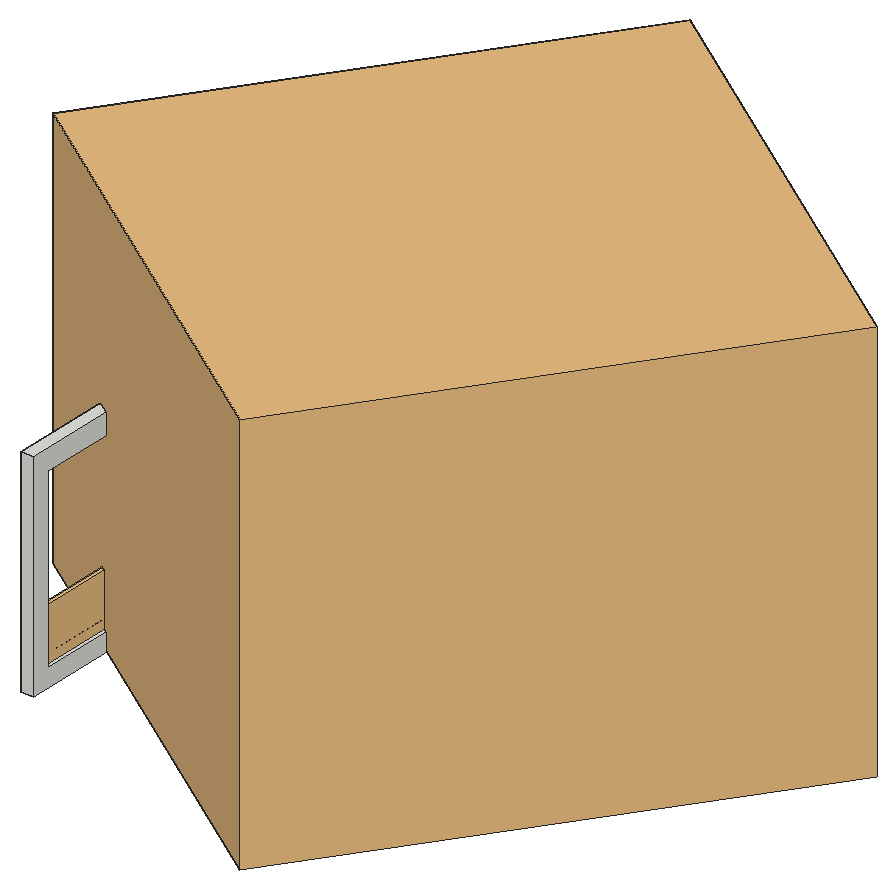
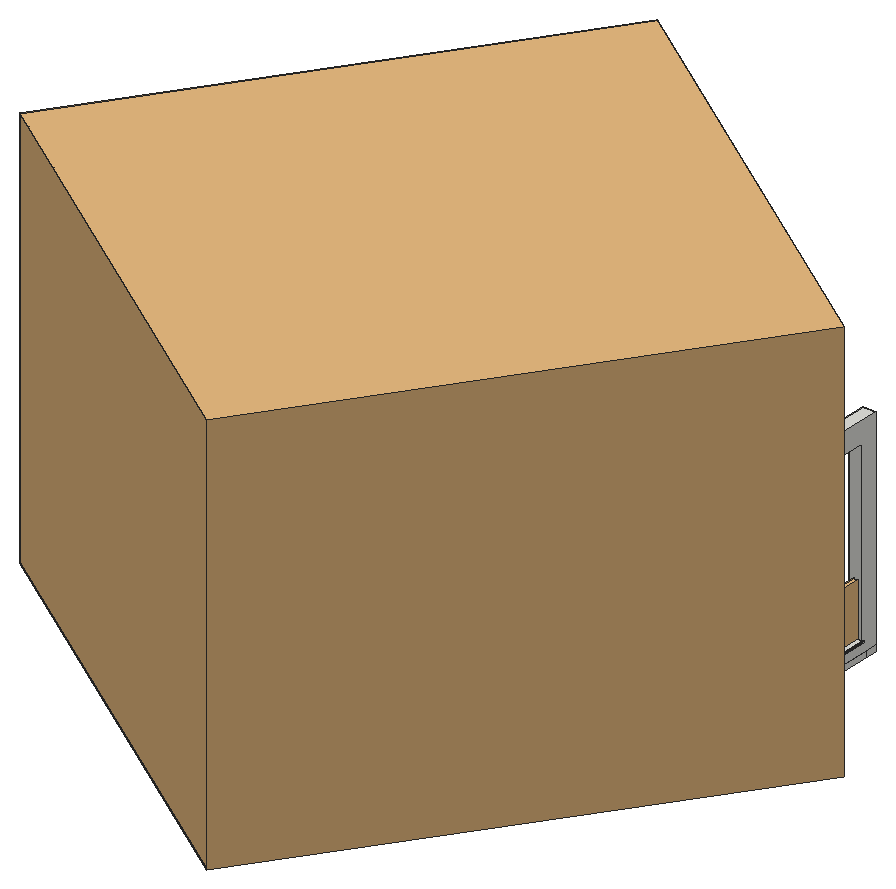
# SketchUp Ruby script. Lengths in inches.
U = 1.inch
M = Sketchup.active_model
def pt(a) = Geom::Point3d.new(a.map { |v| v * U })
def face(e, loops, mat)
  f = e.add_face(loops[0].map { |a| pt(a) })
  loops[1..].each { |l| e.add_face(l.map { |a| pt(a) }).erase! }
  f.material = f.back_material = mat if mat
  f
end
# faces: each face lists its corners as indices into pts; further lists are holes
def faces(e, pts, list, mat = nil) = list.each { |f| face(e, (f[0].is_a?(Array) ? f : [f]).map { |l| l.map { |i| pts[i] } }, mat) }
# xy, xz, yz: faces in a plane at the given z, y or x. An outline is a flat list of corners, or four numbers for a rectangle; further outlines are holes
def ring(l) = l.size == 4 ? [[l[0], l[1]], [l[2], l[1]], [l[2], l[3]], [l[0], l[3]]] : l.each_slice(2).to_a
def flat(e, list, mat, &to3) = list.each { |f| face(e, (f[0].is_a?(Array) ? f : [f]).map { |l| ring(l).map { |u, v| to3.(u, v) } }, mat) }
def xy(e, z, list, mat = nil) = flat(e, list, mat) { |x, y| [x, y, z] }
def xz(e, y, list, mat = nil) = flat(e, list, mat) { |x, z| [x, y, z] }
def yz(e, x, list, mat = nil) = flat(e, list, mat) { |y, z| [x, y, z] }
def lines(e, pts, list) = list.each { |a, b| e.add_line(pt(pts[a]), pt(pts[b])) }
# prism: a flat outline (further loops are holes) pulled along v
def prism(e, loops, v, mat = nil)
  f = face(e, loops, mat); d = Geom::Vector3d.new(v.map { |x| x * U })
  f.pushpull(f.normal.samedirection?(d) ? d.length : -d.length)
end
def box(e, o, s, mat = nil) = prism(e, [[o, [o[0] + s[0], o[1], o[2]], [o[0] + s[0], o[1] + s[1], o[2]], [o[0], o[1] + s[1], o[2]]]], [0, 0, s[2]], mat)
def at(x, y, z, deg = 0) = Geom::Transformation.translation(pt([x, y, z])) * Geom::Transformation.rotation(ORIGIN, Z_AXIS, deg.degrees)
def axes(o, x, y, z) = Geom::Transformation.new([*x, 0, *y, 0, *z, 0, *pt(o).to_a, 1])
def part(name) = M.definitions.add(name)
# library, detail: a bought-in or finely detailed component or shape, given as its bounding box
def library(name, o, s) = part(name).tap { |d| box(d.entities, o, s) }
def detail(e, o, s) = box(e.add_group.entities, o, s)
def put(e, d, t, mat = nil) = e.add_instance(d, t).tap { |i| i.material = mat if mat }
def group(e, t, mat = nil) = e.add_group.tap { |g| g.transformation = t; g.material = mat if mat }.entities
root = M.entities
M.materials.add("[Color M06]").color = [86, 86, 86]
M.materials.add("[Vegetation Blur 03]").color = [83, 114, 18]
c1 = part("ivy")
xy(c1.entities,0,[[0.782,0,0.786,0,0.787,0.005,0.789,0.009,0.821,0.072,0.875,0.147,1.001,0.272,1.073,0.331,1.137,0.363,1.178,0.379,1.223,0.384,1.272,0.383,1.311,0.374,1.36,0.355,1.399,0.334,1.491,0.285,1.541,0.244,1.583,0.199,1.617,0.15,1.64,0.128,1.662,0.115,1.717,0.105,1.745,0.093,1.784,0.054,1.819,0.057,1.854,0.064,1.882,0.075,1.896,0.074,1.91,0.071,1.937,0.063,1.964,0.053,1.99,0.038,2.016,0.015,2.034,0.002,2.04,0,2.038,0.003,2.036,0.007,2.033,0.038,2.036,0.068,2.045,0.1,2.055,0.116,2.064,0.123,2.077,0.129,2.088,0.129,2.106,0.132,2.118,0.13,2.179,0.132,2.207,0.133,2.225,0.133,2.242,0.138,2.22,0.162,2.207,0.186,2.206,0.213,2.212,0.236,2.228,0.262,2.247,0.274,2.298,0.283,2.355,0.294,2.37,0.296,2.376,0.295,2.377,0.3,2.377,0.303,2.385,0.329,2.411,0.37,2.426,0.392,2.449,0.407,2.511,0.426,2.561,0.444,2.619,0.466,2.589,0.469,2.561,0.476,2.501,0.5,2.449,0.516,2.424,0.523,2.401,0.535,2.377,0.556,2.372,0.568,2.36,0.575,2.268,0.586,2.225,0.592,2.207,0.599,2.194,0.61,2.143,0.65,2.13,0.664,2.122,0.682,2.123,0.7,2.13,0.719,2.148,0.75,2.17,0.781,2.195,0.807,2.221,0.828,2.284,0.874,2.291,0.88,2.288,0.887,2.276,0.9,2.267,0.916,2.265,0.933,2.273,0.967,2.292,1.002,2.313,1.03,2.334,1.054,2.348,1.067,2.358,1.074,2.363,1.076,2.362,1.081,2.35,1.094,2.347,1.11,2.35,1.143,2.359,1.18,2.385,1.254,2.415,1.324,2.448,1.393,2.45,1.4,2.446,1.398,2.44,1.394,2.427,1.383,2.402,1.36,2.376,1.339,2.345,1.324,2.305,1.309,2.282,1.303,2.273,1.306,2.245,1.294,2.212,1.287,2.187,1.291,2.163,1.301,2.142,1.316,2.134,1.327,2.124,1.325,2.09,1.292,2.053,1.259,2.014,1.234,1.973,1.215,1.954,1.21,1.931,1.208,1.909,1.212,1.893,1.22,1.879,1.233,1.872,1.248,1.867,1.281,1.864,1.319,1.821,1.258,1.773,1.197,1.726,1.141,1.698,1.121,1.679,1.116,1.666,1.117,1.647,1.122,1.632,1.129,1.62,1.141,1.617,1.154,1.617,1.219,1.621,1.254,1.623,1.268,1.623,1.281,1.618,1.314,1.606,1.346,1.603,1.375,1.607,1.403,1.603,1.467,1.599,1.499,1.605,1.525,1.614,1.552,1.629,1.577,1.635,1.589,1.629,1.587,1.618,1.582,1.596,1.566,1.581,1.556,1.568,1.552,1.557,1.55,1.545,1.553,1.531,1.562,1.522,1.572,1.504,1.591,1.486,1.611,1.474,1.631,1.457,1.666,1.455,1.684,1.457,1.698,1.452,1.715,1.444,1.728,1.424,1.754,1.419,1.772,1.423,1.786,1.434,1.819,1.444,1.848,1.446,1.855,1.44,1.861,1.43,1.867,1.386,1.904,1.349,1.948,1.326,1.973,1.31,1.995,1.288,2.048,1.284,2.153,1.287,2.254,1.284,2.255,1.282,2.253,1.278,2.247,1.274,2.237,1.266,2.216,1.226,2.125,1.208,2.076,1.184,2.033,1.155,1.984,1.135,1.942,1.111,1.899,1.083,1.861,1.053,1.85,1.059,1.83,1.061,1.809,1.056,1.79,1.049,1.767,1.04,1.749,1.018,1.733,0.994,1.726,0.942,1.734,0.95,1.6875,0.944,1.645,0.932,1.608,0.911,1.585,0.881,1.58,0.854,1.582,0.828,1.588,0.785,1.618,0.773,1.625,0.775,1.614,0.779,1.598,0.796,1.502,0.818,1.402,0.861,1.283,0.882,1.224,0.894,1.174,0.892,1.148,0.886,1.123,0.881,1.107,0.872,1.099,0.849,1.094,0.818,1.092,0.789,1.098,0.762,1.107,0.753,1.113,0.721,1.139,0.698,1.163,0.678,1.194,0.665,1.224,0.628,1.28,0.612,1.312,0.606,1.327,0.606,1.314,0.599,1.282,0.594,1.267,0.581,1.256,0.544,1.245,0.512,1.244,0.473,1.249,0.444,1.256,0.382,1.288,0.339,1.306,0.324,1.316,0.317,1.324,0.309,1.326,0.27,1.314,0.227,1.313,0.185,1.3125,0.152,1.317,0.122,1.328,0.092,1.345,0.073,1.353,0.079,1.338,0.092,1.308,0.117,1.249,0.13,1.215,0.139,1.164,0.147,1.148,0.157,1.136,0.163,1.122,0.174,1.086,0.177,1.067,0.182,1.054,0.186,1.043,0.191,1.038,0.211,1.028,0.237,1.005,0.25,0.974,0.253,0.96,0.25,0.944,0.242,0.914,0.243,0.906,0.249,0.902,0.26,0.894,0.289,0.88,0.307,0.873,0.322,0.862,0.364,0.799,0.403,0.738,0.431,0.709,0.439,0.691,0.441,0.678,0.4375,0.66,0.428,0.645,0.394,0.623,0.303,0.594,0.255,0.581,0.214,0.577,0.179,0.573,0.173,0.568,0.175,0.561,0.167,0.55,0.141,0.523,0.113,0.503,0.077,0.49,0.045,0.486,0.026,0.485,0.019,0.486,0.011,0.483,0,0.471,0.014,0.467,0.044,0.455,0.058,0.447,0.07,0.438,0.097,0.411,0.125,0.394,0.158,0.377,0.174,0.366,0.182,0.359,0.185,0.361,0.242,0.331,0.253,0.316,0.258,0.303,0.262,0.283,0.274,0.278,0.308,0.274,0.341,0.252,0.366,0.226,0.366,0.222,0.37,0.22,0.38,0.221,0.395,0.221,0.425,0.216,0.45,0.207,0.465,0.192,0.473,0.178,0.484,0.15,0.489,0.116,0.483,0.089,0.468,0.058,0.45,0.035,0.435,0.018,0.429,0.011,0.434,0.012,0.438,0.014,0.469,0.019,0.542,0.016,0.581,0.015,0.612,0.027,0.68,0.055,0.696,0.057,0.712,0.052,0.73,0.045,0.741,0.036,0.766,0.014]])
c2 = library("Group\#5",[0,0,0],[2.76,154.36,36])
c3 = library("Group\#120",[-119.05,-69.46,2.35],[235.95,219.88,209.78])
c4 = library("Group1",[-41.49,-23.62,0.95],[81.7,76.51,69.13])
c5 = part("Agrupar\#4")
put(c5.entities,c3,axes([132.6,77.36,-2.62],[1.11384,0,0],[0,1.11384,0],[0,0,1.11384]))
put(c5.entities,c4,axes([16.57,9.67,-0.33],[0.3937,0,0],[0,0.3937,0],[0,0,0.3937]))
p = [[139,12,16],[139,12,15],[184.625,93.125,19.69],[184.625,93.125,21.65],[138,174.6,46.56],[137.92,174.6,46.56]]
lines(root,p,[[0,1],[2,3],[4,5]])
put(root,c1,axes([134.05,173.8,27.08],[0.46711,-0.27655,-0.25561],[-0.31156,0.09667,-0.39569],[-0.13813,-1.15324,0.02812]),"[Vegetation Blur 03]")
put(root,c1,axes([133.86,173.8,43.86],[0.29162,-0.09248,0.04712],[0.06325,0.07335,-0.23812],[-0.03677,-0.60733,-0.03593]),"[Vegetation Blur 03]")
put(root,c1,axes([133.625,173.8,15.95],[0.20869,-0.00294,0.30527],[0.37402,-0.00987,-0.17032],[-0.00489,-0.88135,0.00089]),"[Vegetation Blur 03]")
put(root,c1,axes([133.79,173.8,26.5625],[0.11578,-0.07742,0.31422],[0.36947,-0.22297,-0.09932],[-0.11465,-0.79672,-0.00274]),"[Vegetation Blur 03]")
put(root,c1,axes([133.34,173.8,40.79],[0.38841,-0.03974,0.39058],[0.47889,0.01108,-0.31703],[-0.00798,-1.26829,-0.01501]),"[Vegetation Blur 03]")
put(root,c1,axes([134.14,173.8,41.65],[0.29613,-0.07388,-0.10232],[-0.12287,0.05638,-0.24327],[-0.04369,-0.65932,-0.00934]),"[Vegetation Blur 03]")
put(root,c1,axes([134.625,173.8,11.11],[0.14128,-0.20319,-0.29587],[-0.36071,0.14973,-0.1309],[-0.10517,-0.78653,0.05152]),"[Vegetation Blur 03]")
put(root,c1,axes([134.36,173.8,47.71],[0.23115,-0.1069,-0.165],[-0.20647,-0.0259,-0.19002],[-0.03067,-0.63139,0.03573]),"[Vegetation Blur 03]")
put(root,c1,axes([134.67,173.8,30.21],[0.08326,0.10722,-0.24971],[-0.31037,0.02564,-0.0672],[0.00148,-0.65202,-0.0437]),"[Vegetation Blur 03]")
put(root,c1,axes([134.07,173.8,8.57],[0.42261,-0.28747,-0.1193],[-0.16204,-0.06467,-0.35783],[-0.12093,-0.91792,0.06257]),"[Vegetation Blur 03]")
put(root,c1,axes([133.74,173.8,11.61],[0.11289,-0.08937,0.40816],[0.50197,0.01041,-0.09212],[-0.00461,-1.05497,-0.03549]),"[Vegetation Blur 03]")
put(root,c1,axes([134.73,173.8,27.94],[0.13432,-0.12713,-0.31462],[-0.38869,0.03529,-0.11278],[-0.03669,-0.83931,0.04291]),"[Vegetation Blur 03]")
put(root,c1,axes([134.17,173.8,42.74],[0.29319,-0.08212,-0.05398],[-0.06371,0.04494,-0.24127],[-0.04367,-0.61685,-0.01039]),"[Vegetation Blur 03]")
put(root,c1,axes([133.86,173.8,23.81],[0.27283,0.0757,0.1916],[0.23721,-0.13013,-0.2169],[-0.01401,-0.72914,0.0586]),"[Vegetation Blur 03]")
put(root,c1,axes([133.64,173.8,27.48],[0.52424,-0.12738,0.15619],[0.18843,-0.07357,-0.4307],[-0.07036,-1.14606,0.01029]),"[Vegetation Blur 03]")
put(root,c1,axes([134.64,173.8,33.78],[0.19574,-0.01438,-0.25163],[-0.30815,-0.03945,-0.1593],[0.01245,-0.75048,0.0132]),"[Vegetation Blur 03]")
put(root,c1,axes([134.41,173.8,9.83],[0.47968,0.02946,-0.35016],[-0.4281,-0.06549,-0.39149],[0.03188,-1.32271,0.01158]),"[Vegetation Blur 03]")
put(root,c1,axes([134.91,173.8,36.9],[0.09556,-0.13792,-0.34176],[-0.41905,0.10501,-0.08471],[-0.06516,-0.87761,0.04357]),"[Vegetation Blur 03]")
put(root,c1,axes([134.05,173.8,26.375],[0.34163,-0.14558,0.05444],[0.07406,0.06471,-0.28235],[-0.063,-0.71335,-0.03672]),"[Vegetation Blur 03]")
put(root,c1,axes([133.85,173.8,36.14],[0.2559,0.03571,0.2999],[0.36108,-0.20047,-0.20147],[-0.07032,-0.89939,0.05682]),"[Vegetation Blur 03]")
put(root,c1,axes([134.51,173.8,12.26],[0.31122,-0.06083,-0.21678],[-0.26689,-0.02709,-0.25402],[-0.01391,-0.84152,0.02385]),"[Vegetation Blur 03]")
put(root,c1,axes([134.66,173.8,8.21],[0.24157,-0.07416,-0.2538],[-0.31175,0.01688,-0.19842],[-0.02861,-0.81014,0.0191]),"[Vegetation Blur 03]")
put(root,c1,axes([133.86,173.8,35.19],[0.40086,-0.0573,0.17483],[0.21594,0.13183,-0.32299],[0.00594,-0.92596,-0.0568]),"[Vegetation Blur 03]")
put(root,c1,axes([134.16,173.8,42.23],[0.11718,-0.12684,0.22641],[0.28293,-0.00575,-0.09804],[-0.02661,-0.61967,-0.04543]),"[Vegetation Blur 03]")
put(root,c1,axes([134.07,173.8,25.18],[0.52679,-0.06661,-0.07919],[-0.09633,0.02908,-0.43069],[-0.03439,-1.10187,-0.00658]),"[Vegetation Blur 03]")
put(root,c1,axes([133.96,173.8,28.92],[0.52102,-0.20474,0.04178],[0.03433,-0.18504,-0.42777],[-0.1065,-1.06132,0.06652]),"[Vegetation Blur 03]")
put(root,c1,axes([135.05,173.8,14.77],[0.05013,-0.17245,-0.31461],[-0.38087,0.18721,-0.05657],[-0.1028,-0.77773,0.05615]),"[Vegetation Blur 03]")
put(root,c1,axes([134.26,173.8,6.99],[0.48428,-0.17048,-0.13656],[-0.17611,-0.0992,-0.39652],[-0.06201,-1.04969,0.05965]),"[Vegetation Blur 03]")
put(root,c1,axes([133.75,173.8,28.59],[0.31137,-0.19726,0.4006],[0.48849,-0.13513,-0.26337],[-0.10722,-1.1885,-0.03655]),"[Vegetation Blur 03]")
put(root,c1,axes([135.15,173.8,11.78],[0.15704,0.2136,-0.46973],[-0.57168,0.3147,-0.1048],[-0.12334,-1.18664,-0.11235]),"[Vegetation Blur 03]")
put(root,c1,axes([134.75,173.8,10.8],[0.21308,-0.10262,-0.22404],[-0.27243,0.07685,-0.17812],[-0.0602,-0.71097,0.01308]),"[Vegetation Blur 03]")
put(root,c1,axes([135.07,173.8,18.47],[0.09612,-0.08439,-0.33414],[-0.40558,0.12635,-0.08273],[-0.06933,-0.85613,0.02072]),"[Vegetation Blur 03]")
put(root,c1,axes([135.08,173.8,25.61],[0.20248,0.05039,-0.42079],[-0.51446,0.11243,-0.16277],[-0.042,-1.13431,-0.03483]),"[Vegetation Blur 03]")
put(root,c1,axes([134.16,173.8,37.32],[0.06821,0.02412,0.38984],[0.47536,-0.1037,-0.05439],[-0.04826,-0.98747,0.01524]),"[Vegetation Blur 03]")
put(root,c1,axes([134.02,173.8,48.75],[0.24867,-0.15858,0.33537],[0.40835,-0.11898,-0.21053],[-0.08971,-0.98119,-0.02867]),"[Vegetation Blur 03]")
put(root,c1,axes([135.08,173.8,29.97],[0.16222,0.03807,-0.33908],[-0.41557,-0.02093,-0.13279],[0.01621,-0.91758,-0.01104]),"[Vegetation Blur 03]")
put(root,c1,axes([133.83,173.8,11.83],[0.38921,-0.01895,0.37093],[0.44943,-0.16908,-0.31546],[-0.06835,-1.21968,0.03797]),"[Vegetation Blur 03]")
put(root,c1,axes([135.125,173.8,37.18],[0.08292,0.05054,-0.29306],[-0.34577,0.22171,-0.05915],[-0.09993,-0.72524,-0.0385]),"[Vegetation Blur 03]")
put(root,c1,axes([134.95,173.8,22.22],[0.33518,0.12814,-0.38098],[-0.46864,0.20726,-0.26366],[-0.04654,-1.16428,-0.08887]),"[Vegetation Blur 03]")
put(root,c1,axes([135.03,173.8,43.36],[0.33503,-0.17484,-0.44401],[-0.53885,0.1655,-0.28108],[-0.11328,-1.30432,0.02385]),"[Vegetation Blur 03]")
put(root,c1,axes([134.18,173.8,25.04],[0.31064,-0.27454,0.24989],[0.28954,-0.20759,-0.27561],[-0.1665,-0.87322,-0.01304]),"[Vegetation Blur 03]")
put(root,c1,axes([135.45,173.8,25.03],[0.10156,-0.07064,-0.4993],[-0.59327,0.30784,-0.08723],[-0.15326,-1.23847,0.0068]),"[Vegetation Blur 03]")
put(root,c1,axes([134.55,173.8,44.1],[0.37183,-0.05449,-0.06268],[-0.07386,0.08152,-0.30299],[-0.03383,-0.77703,-0.02739]),"[Vegetation Blur 03]")
put(root,c1,axes([135.18,173.8,21.5],[0.29364,-0.08887,-0.43973],[-0.53794,0.07502,-0.24166],[-0.05272,-1.26047,0.01662]),"[Vegetation Blur 03]")
put(root,c1,axes([134.56,173.8,13.67],[0.05383,0.00628,0.24765],[0.29967,-0.10102,-0.04299],[-0.04781,-0.62607,0.00942]),"[Vegetation Blur 03]")
put(root,c1,axes([135.04,173.8,38.52],[0.25146,0.10077,-0.27244],[-0.33679,0.12568,-0.19974],[-0.01997,-0.85077,-0.06178]),"[Vegetation Blur 03]")
put(root,c1,axes([134.86,173.8,39.57],[0.45075,-0.16208,-0.3284],[-0.40131,0.07789,-0.37294],[-0.08406,-1.24093,0.01948]),"[Vegetation Blur 03]")
put(root,c1,axes([134.16,173.8,9.62],[0.59208,-0.24793,0.06374],[0.06017,-0.19072,-0.48897],[-0.13036,-1.21404,0.0638]),"[Vegetation Blur 03]")
put(root,c1,axes([134.48,173.8,15.97],[0.19108,-0.09038,0.20852],[0.25839,0.11931,-0.14958],[0.021,-0.6456,-0.05683]),"[Vegetation Blur 03]")
put(root,c1,axes([134.39,173.8,36.73],[0.36627,-0.13941,0.12421],[0.13945,-0.15724,-0.30166],[-0.09113,-0.8009,0.0376]),"[Vegetation Blur 03]")
put(root,c1,axes([134.95,173.8,37.79],[0.23501,-0.07019,-0.1629],[-0.19555,0.08472,-0.19365],[-0.05258,-0.62881,-0.00791]),"[Vegetation Blur 03]")
put(root,c1,axes([134.46,173.8,17.14],[0.25479,-0.12423,0.18023],[0.21133,-0.13383,-0.2135],[-0.08804,-0.68079,0.00908]),"[Vegetation Blur 03]")
put(root,c1,axes([134.875,173.8,23.66],[0.37161,-0.21861,-0.25288],[-0.28876,0.23657,-0.31481],[-0.15463,-0.96714,-0.01984]),"[Vegetation Blur 03]")
put(root,c1,axes([134.51,173.8,8.28],[0.2775,-0.12673,0.11481],[0.14869,0.07236,-0.22682],[-0.03837,-0.63611,-0.04867]),"[Vegetation Blur 03]")
put(root,c1,axes([135.21,173.8,48.4],[0.21316,0.03069,-0.31446],[-0.38542,0.04396,-0.17335],[-0.01149,-0.90506,-0.01908]),"[Vegetation Blur 03]")
put(root,c1,axes([135.13,173.8,34.06],[0.16581,-0.12598,-0.20066],[-0.24842,0.03821,-0.1405],[-0.04988,-0.60905,0.03269]),"[Vegetation Blur 03]")
put(root,c1,axes([135.31,173.8,19.84],[0.20676,-0.07941,-0.38547],[-0.44776,0.31453,-0.17016],[-0.15519,-1.01328,-0.02261]),"[Vegetation Blur 03]")
put(root,c1,axes([135.04,173.8,33.8],[0.3273,-0.0909,-0.29956],[-0.34726,0.27044,-0.26563],[-0.12681,-0.97518,-0.04574]),"[Vegetation Blur 03]")
put(root,c1,axes([134.82,173.8,31.63],[0.43303,-0.27941,-0.22313],[-0.26455,0.14367,-0.37028],[-0.1523,-1.044,0.00876]),"[Vegetation Blur 03]")
put(root,c1,axes([134.73,173.8,11.71],[0.5589,-0.19272,-0.25961],[-0.28238,0.39595,-0.45114],[-0.17385,-1.26271,-0.10184]),"[Vegetation Blur 03]")
put(root,c1,axes([134.82,173.8,28.42],[0.33014,-0.06379,-0.05513],[-0.06679,0.02302,-0.2706],[-0.03261,-0.69306,-0.00391]),"[Vegetation Blur 03]")
put(root,c1,axes([134.7,173.8,13.71],[0.13106,0.04715,0.22271],[0.27208,-0.09295,-0.10355],[-0.03102,-0.61597,0.03267]),"[Vegetation Blur 03]")
put(root,c1,axes([134.68,173.8,34.65],[0.34203,-0.05341,0.04309],[0.05121,-0.04542,-0.27956],[-0.02898,-0.71072,0.01463]),"[Vegetation Blur 03]")
put(root,c1,axes([134.9,173.8,48.8125],[0.33694,0.0048,-0.1079],[-0.13035,-0.11296,-0.27192],[0.0222,-0.7362,0.04102]),"[Vegetation Blur 03]")
put(root,c1,axes([134.7,173.8,27.48],[0.09035,0.0602,0.28294],[0.33236,-0.23291,-0.06289],[-0.10289,-0.69949,0.04529]),"[Vegetation Blur 03]")
put(root,c1,axes([135.15,173.8,17.49],[0.26178,-0.07777,-0.19292],[-0.23918,-0.11506,-0.20887],[0.01,-0.71663,0.05447]),"[Vegetation Blur 03]")
put(root,c1,axes([134.4,173.8,23.55],[0.46252,-0.08041,0.20679],[0.23593,-0.28736,-0.36906],[-0.10033,-1.0465,0.08545]),"[Vegetation Blur 03]")
put(root,c1,axes([134.61,173.8,18.91],[0.41222,0.08825,0.09854],[0.12607,-0.1297,-0.333],[0.02291,-0.87434,0.05934]),"[Vegetation Blur 03]")
put(root,c1,axes([134.51,173.8,21.91],[0.09143,0.21564,0.47102],[0.58317,-0.16267,-0.06368],[-0.06308,-1.19139,0.09395]),"[Vegetation Blur 03]")
put(root,c1,axes([135.2,173.8,17.27],[0.3587,-0.08547,-0.26789],[-0.31864,0.17898,-0.29317],[-0.08908,-0.98439,-0.03004]),"[Vegetation Blur 03]")
put(root,c1,axes([134.95,173.8,36.04],[0.46854,-0.05722,-0.15501],[-0.19159,-0.07548,-0.38134],[-0.0119,-1.03762,0.03629]),"[Vegetation Blur 03]")
put(root,c1,axes([135.28,173.8,12.8],[0.31159,-0.10577,-0.25159],[-0.29051,0.23223,-0.255],[-0.11522,-0.87155,-0.03742]),"[Vegetation Blur 03]")
put(root,c1,axes([134.7,173.8,46.8],[0.3823,-0.12513,0.1329],[0.15394,-0.13225,-0.31454],[-0.08072,-0.8448,0.02956]),"[Vegetation Blur 03]")
put(root,c1,axes([134.5,173.8,47.86],[0.15219,-0.0035,0.49259],[0.60198,0.09401,-0.12377],[0.04388,-1.27745,-0.01046]),"[Vegetation Blur 03]")
put(root,c1,axes([134.85,173.8,34.125],[0.08947,-0.09548,0.30203],[0.3696,-0.08246,-0.07703],[-0.05008,-0.77914,-0.02886]),"[Vegetation Blur 03]")
put(root,c1,axes([135.43,173.8,8.15],[0.33567,-0.36714,-0.32626],[-0.40941,0.10373,-0.29893],[-0.15499,-1.06915,0.08303]),"[Vegetation Blur 03]")
put(root,c1,axes([135.24,173.8,46.33],[0.49914,0.06889,-0.35402],[-0.43405,0.1716,-0.40237],[-0.0297,-1.34994,-0.06922]),"[Vegetation Blur 03]")
put(root,c1,axes([134.52,173.8,28.58],[0.64177,-0.16774,0.0763],[0.07979,-0.21804,-0.52237],[-0.09498,-1.31665,0.07678]),"[Vegetation Blur 03]")
put(root,c1,axes([135.88,173.8,39.19],[0.20681,0.14961,-0.50522],[-0.62308,0.08477,-0.16594],[-0.01632,-1.34039,-0.06689]),"[Vegetation Blur 03]")
put(root,c1,axes([134.96,173.8,25.4],[0.23912,-0.07387,0.13682],[0.16931,0.00875,-0.19635],[-0.02693,-0.60087,-0.01968]),"[Vegetation Blur 03]")
put(root,c1,axes([134.72,173.8,12.95],[0.10403,0.04174,0.45584],[0.55849,-0.05312,-0.08413],[-0.02168,-1.16792,0.02012]),"[Vegetation Blur 03]")
put(root,c1,axes([135.27,173.8,16.82],[0.41939,0.05909,-0.24373],[-0.29711,-0.06483,-0.343],[0.04165,-1.05748,0.00741]),"[Vegetation Blur 03]")
put(root,c1,axes([134.95,173.8,37.9],[0.15956,0.10306,0.24419],[0.30313,-0.02658,-0.13017],[0.01203,-0.69728,0.04105]),"[Vegetation Blur 03]")
put(root,c1,axes([134.86,173.8,44.42],[0.59182,-0.28218,-0.07799],[-0.07654,0.18572,-0.49252],[-0.14859,-1.21956,-0.05695]),"[Vegetation Blur 03]")
put(root,c1,axes([135.4375,173.8,6.625],[0.26116,-0.07939,-0.16142],[-0.20062,-0.0401,-0.21311],[-0.01886,-0.67295,0.03174]),"[Vegetation Blur 03]")
put(root,c1,axes([135.16,173.8,13.1875],[0.45644,-0.12973,-0.15733],[-0.18474,0.13729,-0.3748],[-0.08372,-1.01031,-0.03073]),"[Vegetation Blur 03]")
put(root,c1,axes([134.87,173.8,34.54],[0.32504,0.10399,0.20827],[0.26014,-0.12611,-0.26052],[0.00118,-0.84097,0.06482]),"[Vegetation Blur 03]")
put(root,c1,axes([135.61,173.8,43.73],[0.44413,0.17265,-0.41061],[-0.51006,0.15289,-0.35736],[-0.00095,-1.3725,-0.09146]),"[Vegetation Blur 03]")
put(root,c1,axes([135.22,173.8,9.05],[0.5663,-0.16171,-0.26651],[-0.30497,0.30432,-0.46069],[-0.14072,-1.31032,-0.0741]),"[Vegetation Blur 03]")
put(root,c1,axes([135.45,173.8,24.29],[0.32555,-0.21056,-0.17248],[-0.21105,0.06347,-0.27751],[-0.10292,-0.79617,0.02349]),"[Vegetation Blur 03]")
put(root,c1,axes([134.76,173.8,14.29],[0.35259,-0.1904,0.31199],[0.38853,0.00444,-0.29204],[-0.06112,-1.07015,-0.05672]),"[Vegetation Blur 03]")
put(root,c1,axes([136.08,173.8,46.18],[0.12519,-0.10736,-0.42184],[-0.51949,-0.03465,-0.1013],[0.00417,-1.09384,0.04461]),"[Vegetation Blur 03]")
put(root,c1,axes([135.07,173.8,47.92],[0.26564,-0.06538,0.20861],[0.24422,-0.17627,-0.21582],[-0.08188,-0.73784,0.03307]),"[Vegetation Blur 03]")
put(root,c1,axes([134.84,173.8,22.9],[0.57824,-0.2854,0.09144],[0.09076,-0.20234,-0.48162],[-0.15346,-1.19504,0.05971]),"[Vegetation Blur 03]")
put(root,c1,axes([134.66,173.8,36.52],[0.63449,0.08244,0.15008],[0.18708,-0.13099,-0.51549],[0.02055,-1.35306,0.05905]),"[Vegetation Blur 03]")
put(root,c1,axes([135.96,173.8,47.91],[0.1485,0.06744,-0.32773],[-0.39216,0.22625,-0.11103],[-0.09244,-0.8515,-0.05546]),"[Vegetation Blur 03]")
put(root,c1,axes([134.85,173.8,33.63],[0.21618,-0.06557,0.43271],[0.52184,-0.19331,-0.17826],[-0.09899,-1.16227,0.00524]),"[Vegetation Blur 03]")
put(root,c1,axes([134.76,173.8,26.7],[0.61927,-0.03223,0.11526],[0.14207,0.12094,-0.50313],[-0.00213,-1.30144,-0.04961]),"[Vegetation Blur 03]")
put(root,c1,axes([134.66,173.8,23.15],[0.45704,-0.07073,0.34791],[0.42202,-0.13355,-0.37354],[-0.06933,-1.27915,0.01976]),"[Vegetation Blur 03]")
put(root,c1,axes([135.5,173.8,11.85],[0.48214,-0.22782,-0.28181],[-0.31501,0.32234,-0.39997],[-0.17959,-1.177,-0.05499]),"[Vegetation Blur 03]")
put(root,c1,axes([134.97,173.8,21.76],[0.23423,-0.31556,0.37462],[0.44905,-0.24958,-0.22008],[-0.18046,-1.03065,-0.06141]),"[Vegetation Blur 03]")
put(root,c1,axes([135.2,173.8,8.6875],[0.21432,-0.13844,0.2244],[0.28013,0.00181,-0.17803],[-0.04065,-0.71738,-0.04375]),"[Vegetation Blur 03]")
put(root,c1,axes([134.82,173.8,31.27],[0.38223,0.09975,0.36551],[0.44923,0.00523,-0.31313],[0.03341,-1.2116,0.02874]),"[Vegetation Blur 03]")
put(root,c1,axes([135.44,173.8,32.8125],[0.32645,-0.19251,-0.02516],[-0.03795,-0.04316,-0.27603],[-0.0909,-0.67338,0.02489]),"[Vegetation Blur 03]")
put(root,c1,axes([135.32,173.8,44.17],[0.36239,0.03439,0.0325],[0.04011,-0.01114,-0.29602],[0.01602,-0.75014,0.00588]),"[Vegetation Blur 03]")
put(root,c1,axes([135.76,173.8,47.07],[0.31224,-0.04153,-0.22289],[-0.2695,0.10455,-0.25454],[-0.04857,-0.84719,-0.02048]),"[Vegetation Blur 03]")
put(root,c1,axes([134.98,173.8,19.93],[0.19345,-0.03327,0.47278],[0.57353,-0.16922,-0.15818],[-0.0831,-1.24533,0.00886]),"[Vegetation Blur 03]")
put(root,c1,axes([135.18,173.8,48.58],[0.22749,-0.09368,0.31124],[0.37139,-0.17878,-0.18927],[-0.09787,-0.89612,0.00522]),"[Vegetation Blur 03]")
put(root,c1,axes([135.16,173.8,20.41],[0.30062,0.06409,0.25513],[0.31279,-0.14376,-0.23982],[-0.02918,-0.88082,0.05771]),"[Vegetation Blur 03]")
put(root,c1,axes([136.02,173.8,38.62],[0.2286,-0.00259,-0.27195],[-0.33307,0.02295,-0.18652],[-0.00991,-0.83122,-0.0043]),"[Vegetation Blur 03]")
put(root,c1,axes([135.73,173.8,39.75],[0.44457,-0.30415,-0.24459],[-0.31847,-0.07486,-0.37092],[-0.10118,-1.10076,0.09281]),"[Vegetation Blur 03]")
put(root,c1,axes([135.37,173.8,8.98],[0.33883,-0.03876,0.14234],[0.17237,-0.07132,-0.27636],[-0.03256,-0.78094,0.01817]),"[Vegetation Blur 03]")
put(root,c1,axes([135.02,173.8,26.98],[0.53293,-0.19106,0.2627],[0.2994,-0.28671,-0.43737],[-0.15029,-1.24869,0.06023]),"[Vegetation Blur 03]")
put(root,c1,axes([135.75,173.8,44.81],[0.4979,-0.40473,-0.18477],[-0.2554,-0.09899,-0.42431],[-0.15719,-1.12116,0.10416]),"[Vegetation Blur 03]")
put(root,c1,axes([136.45,173.8,45.72],[0.11758,-0.14394,-0.33997],[-0.41694,0.10295,-0.1029],[-0.06765,-0.88473,0.04334]),"[Vegetation Blur 03]")
put(root,c1,axes([135.58,173.8,45.8],[0.42779,-0.01722,0.00276],[0.0027,-0.07154,-0.34805],[-0.00862,-0.87743,0.02832]),"[Vegetation Blur 03]")
put(root,c1,axes([135.46,173.8,35.4],[0.18898,0.02634,0.37085],[0.44381,-0.22984,-0.14807],[-0.09838,-0.98629,0.04441]),"[Vegetation Blur 03]")
put(root,c1,axes([135.4,173.8,12.68],[0.62343,-0.11777,0.0104],[0.0079,-0.1089,-0.50918],[-0.0581,-1.27854,0.04241]),"[Vegetation Blur 03]")
put(root,c1,axes([135.75,173.8,48.62],[0.24814,-0.07421,0.13501],[0.16554,-0.02052,-0.20443],[-0.03556,-0.61336,-0.0095]),"[Vegetation Blur 03]")
put(root,c1,axes([136.1,173.8,48.75],[0.32819,0.01887,-0.10221],[-0.12554,0.06541,-0.2666],[-0.0028,-0.71988,-0.0269]),"[Vegetation Blur 03]")
put(root,c1,axes([135.51,173.8,14.26],[0.31828,-0.32105,0.3684],[0.45752,-0.11523,-0.27908],[-0.137,-1.13071,-0.07616]),"[Vegetation Blur 03]")
put(root,c1,axes([136.17,173.8,49.43],[0.36865,-0.17556,-0.1237],[-0.14943,0.05438,-0.30876],[-0.08901,-0.81841,0.00602]),"[Vegetation Blur 03]")
put(root,c1,axes([136.13,173.8,43.74],[0.30667,-0.21087,0.08542],[0.09735,-0.07998,-0.26385],[-0.10945,-0.662,0.00467]),"[Vegetation Blur 03]")
put(root,c1,axes([135.87,173.8,41.29],[0.29759,0.01634,0.29239],[0.3571,0.0663,-0.24267],[0.02985,-0.95609,-0.01183]),"[Vegetation Blur 03]")
put(root,c1,axes([136.18,173.8,41.7],[0.43208,-0.00485,-0.01137],[-0.01346,0.125,-0.34915],[-0.00429,-0.88078,-0.04949]),"[Vegetation Blur 03]")
put(root,c1,axes([135.97,173.8,46.17],[0.38148,-0.02964,0.33346],[0.3977,-0.23961,-0.3064],[-0.09475,-1.12505,0.05647]),"[Vegetation Blur 03]")
put(root,c1,axes([136.07,173.8,38.58],[0.54527,-0.10858,0.11727],[0.14945,0.14116,-0.4423],[-0.03309,-1.15173,-0.06527]),"[Vegetation Blur 03]")
put(root,c1,axes([135.91,173.8,47.01],[0.28018,-0.09633,0.48866],[0.59963,-0.03141,-0.22997],[-0.03369,-1.35996,-0.0293]),"[Vegetation Blur 03]")
g1 = group(root,at(140,0,4))
xy(g1,0,[[-1,0,-1,9,-1.25,9,-1.25,180,8,180,8,0]])
xy(g1,4,[[-1.25,9,-1,176]])
xy(g1,11,[[-2,12,-1,164]])
xy(g1,11.99,[[-1.65,12,-1.62,164]])
xy(g1,12,[[-1.58,12,-1.54,164],[-1.54,12,-1.5,164],[-1.5,12,8,164]])
xy(g1,132,[[-1,12,8,164],[-1.25,176,-1,180]])
xy(g1,146,[[-1,0,8,180]])
xz(g1,0,[[-1,0,8,146]])
xz(g1,9,[[-1.25,0,-1,4]])
xz(g1,12,[[-2,11,-1,11,-1,12,-1.58,12,-1.62,11.99,-1.65,11.99,-1.6875,11.98,-1.72,11.97,-1.75,11.96,-1.78,11.94,-1.8,11.93,-1.83,11.91,-1.85,11.89,-1.875,11.875,-1.89,11.85,-1.91,11.83,-1.93,11.8,-1.94,11.78,-1.96,11.75,-1.97,11.72,-1.98,11.6875,-1.99,11.65,-1.99,11.62,-2,11.58],[-1,12,8,132]])
xz(g1,164,[[-2,11,-2,11.58,-1.99,11.62,-1.99,11.65,-1.98,11.6875,-1.97,11.72,-1.96,11.75,-1.94,11.78,-1.93,11.8,-1.91,11.83,-1.89,11.85,-1.875,11.875,-1.85,11.89,-1.83,11.91,-1.8,11.93,-1.78,11.94,-1.75,11.96,-1.72,11.97,-1.6875,11.98,-1.65,11.99,-1.62,11.99,-1.58,12,-1,12,-1,11],[-1,12,8,132]])
xz(g1,176,[[-1.25,4,-1,132]])
xz(g1,180,[[-1.25,0,-1.25,132,-1,132,-1,146,8,146,8,0]])
yz(g1,-2,[[12,11,164,11.5],[12,11.5,164,11.54],[12,11.54,164,11.58]])
yz(g1,-1.99,[[12,11.62,164,11.65]])
yz(g1,-1.25,[[9,0,176,4],[176,0,180,132]])
yz(g1,-1,[[0,0,9,4],[[0,4,176,146],[12,11,164,132]],[176,132,180,146]])
yz(g1,8,[[[0,0,180,146],[12,12,164,132]]])
p = [[-1.99,12,11.62],[-1.99,164,11.62],[-2,164,11.58],[-2,12,11.58],[-1.94,12,11.78],[-1.94,164,11.78],
  [-1.96,164,11.75],[-1.96,12,11.75],[-1.97,164,11.72],[-1.97,12,11.72],[-1.98,164,11.6875],[-1.98,12,11.6875],
  [-1.99,164,11.65],[-1.99,12,11.65],[-1.89,12,11.85],[-1.89,164,11.85],[-1.91,164,11.83],[-1.91,12,11.83],
  [-1.93,164,11.8],[-1.93,12,11.8],[-1.875,12,11.875],[-1.875,164,11.875],[-1.83,12,11.91],[-1.83,164,11.91],
  [-1.85,164,11.89],[-1.85,12,11.89],[-1.75,12,11.96],[-1.75,164,11.96],[-1.78,164,11.94],[-1.78,12,11.94],
  [-1.8,164,11.93],[-1.8,12,11.93],[-1.65,12,11.99],[-1.65,164,11.99],[-1.6875,164,11.98],[-1.6875,12,11.98],
  [-1.72,164,11.97],[-1.72,12,11.97],[-1.58,12,12],[-1.58,164,12],[-1.62,164,11.99],[-1.62,12,11.99]]
faces(g1,p,[[0,1,2,3],[4,5,6,7],[7,6,8,9],[9,8,10,11],[11,10,12,13],[14,15,16,17],[17,16,18,19],[19,18,5,4],
  [20,21,15,14],[22,23,24,25],[25,24,21,20],[26,27,28,29],[29,28,30,31],[31,30,23,22],[32,33,34,35],[35,34,36,37],
  [37,36,27,26],[38,39,40,41]])
put(root,c2,axes([142.12,12,16],[1,0,0],[0,0.9847,0],[0,0,1]),"[Color M06]")
put(root,c5,axes([66.82,117.79,5.05],[1.08439,-0.75087,0],[0.82038,1.18477,0],[0,0,1.17334]))
